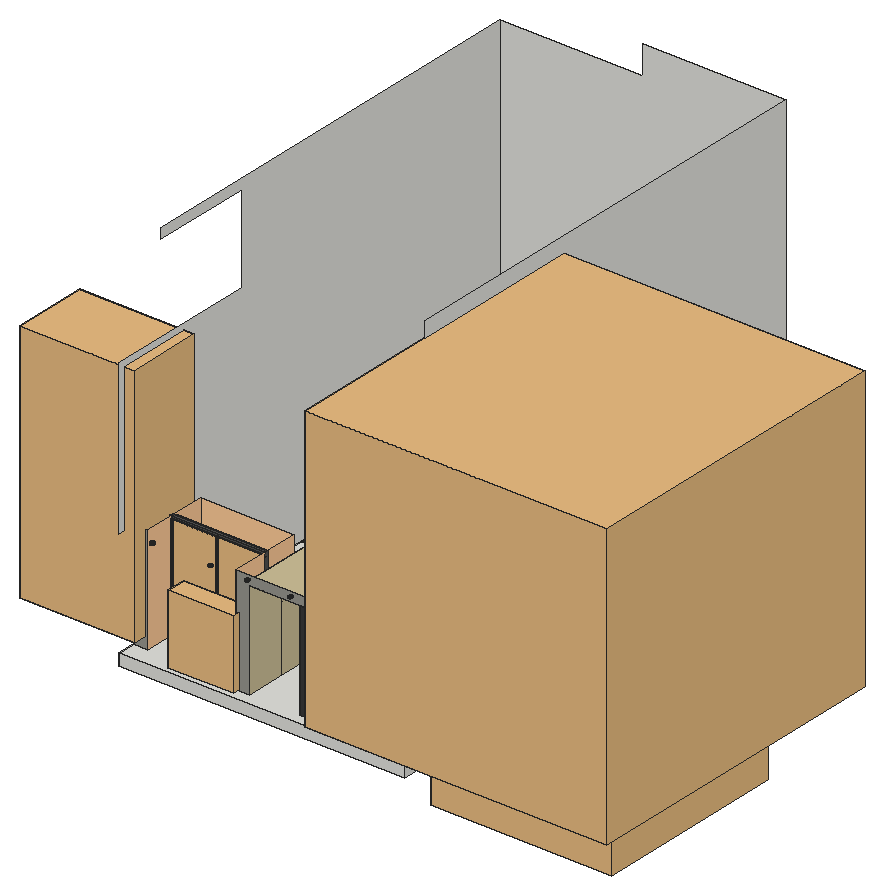
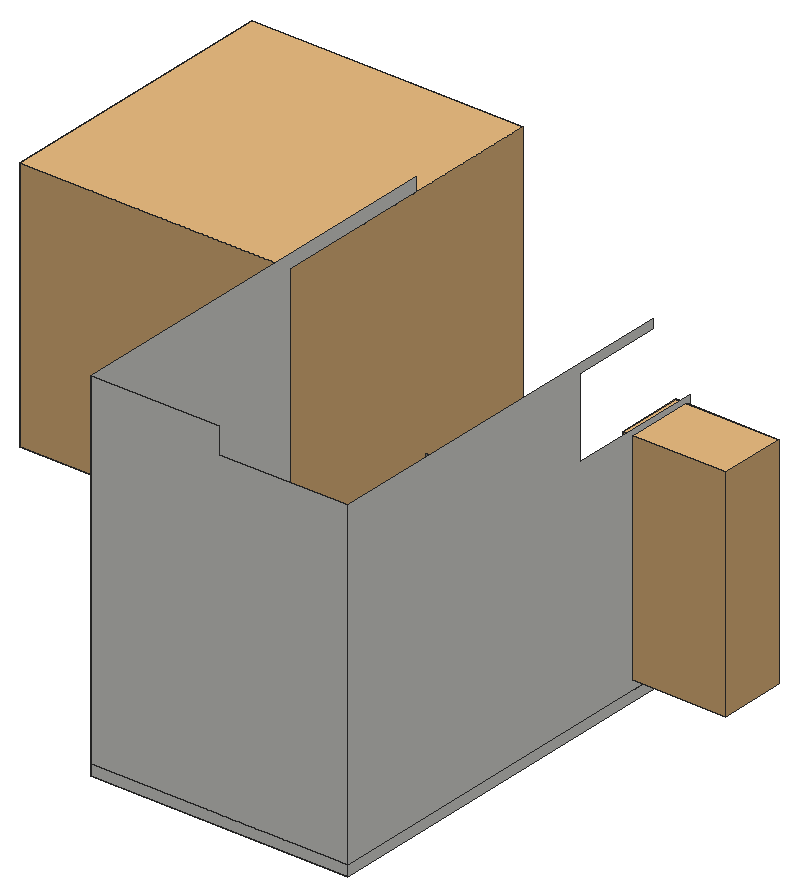
# SketchUp Ruby script. Lengths in inches.
U = 1.inch
M = Sketchup.active_model
def pt(a) = Geom::Point3d.new(a.map { |v| v * U })
def face(e, loops, mat)
  f = e.add_face(loops[0].map { |a| pt(a) })
  loops[1..].each { |l| e.add_face(l.map { |a| pt(a) }).erase! }
  f.material = f.back_material = mat if mat
  f
end
# faces: each face lists its corners as indices into pts; further lists are holes
def faces(e, pts, list, mat = nil) = list.each { |f| face(e, (f[0].is_a?(Array) ? f : [f]).map { |l| l.map { |i| pts[i] } }, mat) }
# xy, xz, yz: faces in a plane at the given z, y or x. An outline is a flat list of corners, or four numbers for a rectangle; further outlines are holes
def ring(l) = l.size == 4 ? [[l[0], l[1]], [l[2], l[1]], [l[2], l[3]], [l[0], l[3]]] : l.each_slice(2).to_a
def flat(e, list, mat, &to3) = list.each { |f| face(e, (f[0].is_a?(Array) ? f : [f]).map { |l| ring(l).map { |u, v| to3.(u, v) } }, mat) }
def xy(e, z, list, mat = nil) = flat(e, list, mat) { |x, y| [x, y, z] }
def xz(e, y, list, mat = nil) = flat(e, list, mat) { |x, z| [x, y, z] }
def yz(e, x, list, mat = nil) = flat(e, list, mat) { |y, z| [x, y, z] }
def lines(e, pts, list) = list.each { |a, b| e.add_line(pt(pts[a]), pt(pts[b])) }
# prism: a flat outline (further loops are holes) pulled along v
def prism(e, loops, v, mat = nil)
  f = face(e, loops, mat); d = Geom::Vector3d.new(v.map { |x| x * U })
  f.pushpull(f.normal.samedirection?(d) ? d.length : -d.length)
end
def box(e, o, s, mat = nil) = prism(e, [[o, [o[0] + s[0], o[1], o[2]], [o[0] + s[0], o[1] + s[1], o[2]], [o[0], o[1] + s[1], o[2]]]], [0, 0, s[2]], mat)
def at(x, y, z, deg = 0) = Geom::Transformation.translation(pt([x, y, z])) * Geom::Transformation.rotation(ORIGIN, Z_AXIS, deg.degrees)
def axes(o, x, y, z) = Geom::Transformation.new([*x, 0, *y, 0, *z, 0, *pt(o).to_a, 1])
def part(name) = M.definitions.add(name)
# library, detail: a bought-in or finely detailed component or shape, given as its bounding box
def library(name, o, s) = part(name).tap { |d| box(d.entities, o, s) }
def detail(e, o, s) = box(e.add_group.entities, o, s)
def put(e, d, t, mat = nil) = e.add_instance(d, t).tap { |i| i.material = mat if mat }
def group(e, t, mat = nil) = e.add_group.tap { |g| g.transformation = t; g.material = mat if mat }.entities
root = M.entities
M.materials.add("AM113_062_Tilia").color = [58, 81, 37]
M.materials.add("AM113_062_Tilia_Bark").color = [88, 85, 72]
M.materials.add("Brick Wall Grey Stone 01 200cm").color = [152, 151, 144]
M.materials.add("Generic").color = [218, 205, 180]
M.materials.add("Glass_Tinted_Gray").color = [0, 0, 0]
M.materials["Glass_Tinted_Gray"].alpha = 0.125
M.materials.add("Wall  Paint Fine Grain 01 Yellow 100cm").color = [207, 193, 153]
M.materials.add("[0135_DarkGray]").color = [81, 81, 81]
M.materials.add("[Color C02]").color = [255, 204, 153]
M.materials.add("[Color E05]").color = [239, 239, 0]
M.materials["[Color E05]"].alpha = 0.89
M.materials.add("[Color M07]").color = [58, 58, 58]
M.materials.add("[Color M08]").color = [30, 30, 30]
M.materials.add("[Granite Dark Gray]").color = [69, 68, 68]
M.materials.add("[Mirror 02]").color = [229, 229, 229]
M.materials.add("[Terrazzo Light Blue]").color = [196, 214, 227]
M.materials.add("[Translucent Glass Gray]").color = [128, 128, 128]
M.materials["[Translucent Glass Gray]"].alpha = 0.5
c1 = library("Curtain set",[0,0,0],[14.46,147.43,135.83])
c2 = part("PENTEK_RP Fineline 50S_Sliding_DoorCase_E1")
box(c2.entities,[0,0,0],[1.51,3.66,99.27],"[0135_DarkGray]")
c3 = part("PENTEK_RP Fineline 50S_SlidingDooe_Case_E2")
box(c3.entities,[0,0,0],[96.25,3.66,1.51],"[0135_DarkGray]")
c4 = part("pentek_RP Fineline 50S_SlidingDoor_Case")
put(c4.entities,c2,at(97.76,0,0))
put(c4.entities,c3,at(1.51,0,0))
put(c4.entities,c2,at(0,0,0))
put(c4.entities,c3,at(1.51,0,97.76))
c5 = part("PENTEK_RP Fineline 50S_SlidingDoor_GlazingBead_2")
box(c5.entities,[0,0,0],[0.56,0.59,94.39],"[0135_DarkGray]")
c6 = part("PENTEK_RP Fineline 50S_SlidingDoor_Glass")
box(c6.entities,[0,0,0],[46.58,0.16,94.39],"Glass_Tinted_Gray")
c7 = part("PENTEK_RP Fineline 50S_SlidingDoor_GlazingBead")
box(c7.entities,[0,0,0],[45.47,0.59,0.56],"[0135_DarkGray]")
c8 = part("PENTEK_RP Fineline 50S_SlidingDoor_Leaf_E1")
xy(c8.entities,0,[[0,0,0.93,1.97],[0.93,1.57,1.49,1.97]],"[0135_DarkGray]")
xy(c8.entities,96.25,[[0,0,0.93,0,0.93,1.57,1.49,1.57,1.49,1.97,0,1.97]],"[0135_DarkGray]")
xz(c8.entities,0,[[0,0,0.93,96.25]],"[0135_DarkGray]")
xz(c8.entities,1.57,[[0.93,0,1.49,95.32],[0.93,95.32,1.49,96.25]],"[0135_DarkGray]")
xz(c8.entities,1.97,[[0,0,1.49,96.25]],"[0135_DarkGray]")
yz(c8.entities,0,[[0,0,1.97,96.25]],"[0135_DarkGray]")
yz(c8.entities,0.93,[[0,0,1.57,0.93],[0,0.93,1.57,95.32],[0,95.32,1.57,96.25]],"[0135_DarkGray]")
yz(c8.entities,1.49,[[1.57,0,1.97,95.32],[1.57,95.32,1.97,96.25]],"[0135_DarkGray]")
c9 = part("PENTEK_RP Fineline 50S_SlidingDoor_Leaf_E2")
xy(c9.entities,0,[[0,0,0,1.57,0.56,1.57,0.56,1.97,46.02,1.97,46.02,1.57,46.58,1.57,46.58,0]],"[0135_DarkGray]")
xy(c9.entities,0.93,[[0,0,46.58,1.57]],"[0135_DarkGray]")
xy(c9.entities,1.49,[[0.56,1.57,46.02,1.97]],"[0135_DarkGray]")
xz(c9.entities,0,[[0,0,46.58,0.93]],"[0135_DarkGray]")
xz(c9.entities,1.57,[[0,0,0.56,0.93],[46.02,0,46.58,0.93],[0.56,0.93,46.02,1.49]],"[0135_DarkGray]")
xz(c9.entities,1.97,[[0.56,0,46.02,1.49]],"[0135_DarkGray]")
yz(c9.entities,0,[[0,0,1.57,0.93]],"[0135_DarkGray]")
yz(c9.entities,0.56,[[1.57,0,1.97,0.93],[1.57,0.93,1.97,1.49]],"[0135_DarkGray]")
yz(c9.entities,46.02,[[1.57,0,1.97,0.93],[1.57,0.93,1.97,1.49]],"[0135_DarkGray]")
yz(c9.entities,46.58,[[0,0,1.57,0.93]],"[0135_DarkGray]")
c10 = part("PENTEK_RP Fineline S_SlidingDoor_Leaf1")
put(c10.entities,c5,at(0.93,0,0.93))
put(c10.entities,c5,at(46.96,0,0.93))
put(c10.entities,c6,at(1.49,1.42,0.93))
put(c10.entities,c7,at(1.49,0,0.93))
put(c10.entities,c6,at(1.49,0.59,0.93),"[Terrazzo Light Blue]")
put(c10.entities,c8,at(0,0,0))
put(c10.entities,c8,axes([48.44,0,0],[-1,0,0],[0,1,0],[0,0,1]))
put(c10.entities,c9,axes([0.93,0,96.25],[1,0,0],[0,1,0],[0,0,-1]))
put(c10.entities,c9,at(0.93,0,0))
put(c10.entities,c7,at(1.49,0,94.77))
c11 = part("PENTEK_RP Fineline 50S_SlidingDoor_Leaf2")
put(c11.entities,c6,at(1.49,1.42,0.93))
put(c11.entities,c7,at(1.49,0,94.77))
put(c11.entities,c5,at(46.96,0,0.93))
put(c11.entities,c6,at(1.49,0.59,0.93),"[Mirror 02]")
put(c11.entities,c5,at(0.93,0,0.93))
put(c11.entities,c8,at(0,0,0))
put(c11.entities,c8,axes([48.44,0,0],[-1,0,0],[0,1,0],[0,0,1]))
put(c11.entities,c7,at(1.49,0,0.93))
put(c11.entities,c9,axes([0.93,0,96.25],[1,0,0],[0,1,0],[0,0,-1]))
put(c11.entities,c9,at(0.93,0,0))
c12 = part("PENTEK - Slimmest Steel Sliding Door / Window\#1")
put(c12.entities,c4,at(0,-1.88,-0.09))
put(c12.entities,c10,at(1.51,-2.27,1.42))
put(c12.entities,c11,at(49.32,-0.3,1.42))
c13 = part("Agrupar\#57")
prism(c13.entities,[[[1.18,24.41,51.97],[1.18,0,51.97],[1.18,0,0],[1.18,24.41,0]],[[1.18,1.57,50.39],[1.18,22.83,50.39],[1.18,22.83,1.57],[1.18,1.57,1.57]]],[-1.18,0,0])
c14 = part("Agrupar\#59")
box(c14.entities,[0,0,0],[0.24,21.26,16.54])
c15 = part("Agrupar\#58")
prism(c15.entities,[[[0,0,0],[0,0,19.69],[0,24.41,19.69],[0,24.41,0]],[[0,1.57,1.57],[0,22.83,1.57],[0,22.83,18.11],[0,1.57,18.11]]],[1.18,0,0])
c16 = part("Agrupar\#56")
box(c16.entities,[0,0,0],[4.72,24.41,1.57])
c17 = part("Agrupar\#55")
prism(c17.entities,[[[0,0,0],[0,0,97.64],[0,27.56,97.64],[0,27.56,0]],[[0,25.98,1.57],[0,25.98,96.0625],[0,1.57,96.0625],[0,1.57,1.57]]],[4.72,0,0])
c18 = part("Agrupar\#60")
box(c18.entities,[0,0,0],[0.24,21.26,48.82])
c19 = part("Janela Maxim ar")
put(c19.entities,c13,at(1.77,1.57,22.83))
put(c19.entities,c14,at(2.36,3.15,77.95),"[Translucent Glass Gray]")
put(c19.entities,c15,at(1.77,1.57,1.57))
put(c19.entities,c16,at(0,1.57,74.8))
put(c19.entities,c16,at(0,1.57,21.26))
put(c19.entities,c15,at(1.77,1.57,76.38))
put(c19.entities,c17,at(0,0,0))
put(c19.entities,c14,at(2.36,3.15,3.15),"[Translucent Glass Gray]")
put(c19.entities,c18,at(2.36,3.15,24.41),"[Translucent Glass Gray]")
c20 = part("Agrupar\#54")
box(c20.entities,[0,0,0],[7.09,27.56,0.79])
c21 = part("JA-70x250")
put(c21.entities,c19,at(2.36,0,0.79),"[Color M08]")
put(c21.entities,c20,at(0,0,0),"[Granite Dark Gray]")
c22 = library("Entrance door assembly",[0,0,0],[51.57,9.61,84.84])
c23 = library("Plant",[-27.84,-31.84,-1.26],[68.28,70.82,154.38])
c24 = library("Group\#7",[0,0,0],[99.27,8.68,96.02])
c25 = library("30",[-486.49,477.14,411.4],[26.62,27.13,73.11])
c26 = library("AM113_062_Tilia_Defintion",[-350.67,-364.73,-2.58],[672.29,726.36,1000])
c27 = library("AM113_062_Tilia_Defintion1",[-524.84,-500,219.37],[933.41,1000,877.77])
c28 = part("Group4\#2")
put(c28.entities,c26,axes([0,0,0],[0.28109,0,0],[0,0.28109,0],[0,0,0.28109]),"AM113_062_Tilia_Bark")
put(c28.entities,c27,axes([0,0,0],[0.33697,0,0],[0,0.33697,0],[0,0,0.33697]),"AM113_062_Tilia")
c29 = part("11")
put(c29.entities,c28,at(1388.71,2.74,19.08))
xy(root,0,[[179.7,11.0625,179.7,207.1875,126.76,207.1875,126.76,54.0625,112.5,54.0625,112.5,88.375,14.7,88.375,14.7,19.125,0,19.125,0,497,299.0625,497,299.0625,12.5,280.68,12.5,280.68,190.6875,189.32,190.6875,189.32,11.0625],[112.5,12.5,126.76,54.0625]])
xy(root,98.74,[[189.32,64.65,280.68,67.0625],[189.32,68.5625,280.68,84.21]])
xy(root,98.74,[[189.32,67.0625,280.68,68.5625]],"[Color E05]")
xy(root,102.36,[[179.7,11.0625,189.32,12.5],[126.76,12.5,179.7,17.9375],[179.7,12.5,189.32,17.9375],[189.32,12.5,280.68,15.9375]])
xy(root,102.36,[[189.32,15.9375,280.68,17.9375]],"[Color E05]")
xy(root,107.49,[[189.32,17.9375,280.68,64.65],[189.32,84.21,280.68,190.6875]])
xy(root,107.49,[[126.76,17.9375,179.7,207.1875]],"Wall  Paint Fine Grain 01 Yellow 100cm")
xy(root,109.8125,[[29.97,4.05,29.45,4.11,28.97,4.3125,28.55,4.63,28.23,5.05,28.03,5.53,27.97,6.05,28.03,6.5625,28.23,7.05,28.55,7.46,28.97,7.78,29.45,7.98,29.97,8.05,30.48,7.98,30.97,7.78,31.38,7.46,31.7,7.05,31.9,6.5625,31.97,6.05,31.9,5.53,31.7,5.05,31.38,4.63,30.97,4.3125,30.48,4.11]])
xy(root,110.68,[[90.97,4.05,90.45,4.11,89.97,4.3125,89.55,4.63,89.23,5.05,89.03,5.53,88.97,6.05,89.03,6.5625,89.23,7.05,89.55,7.46,89.97,7.78,90.45,7.98,90.97,8.05,91.48,7.98,91.97,7.78,92.38,7.46,92.7,7.05,92.9,6.5625,92.97,6.05,92.9,5.53,92.7,5.05,92.38,4.63,91.97,4.3125,91.48,4.11],[129.28,4.05,128.76,4.11,128.28,4.3125,127.86,4.63,127.55,5.05,127.35,5.53,127.28,6.05,127.35,6.5625,127.55,7.05,127.86,7.46,128.28,7.78,128.76,7.98,129.28,8.05,129.8,7.98,130.28,7.78,130.69,7.46,131.01,7.05,131.21,6.5625,131.28,6.05,131.21,5.53,131.01,5.05,130.69,4.63,130.28,4.3125,129.8,4.11],[174.28,4.05,173.76,4.11,173.28,4.3125,172.86,4.63,172.55,5.05,172.35,5.53,172.28,6.05,172.35,6.5625,172.55,7.05,172.86,7.46,173.28,7.78,173.76,7.98,174.28,8.05,174.8,7.98,175.28,7.78,175.69,7.46,176.01,7.05,176.21,6.5625,176.28,6.05,176.21,5.53,176.01,5.05,175.69,4.63,175.28,4.3125,174.8,4.11],[208.4,4.05,207.89,4.11,207.4,4.3125,206.99,4.63,206.67,5.05,206.47,5.53,206.4,6.05,206.47,6.5625,206.67,7.05,206.99,7.46,207.4,7.78,207.89,7.98,208.4,8.05,208.92,7.98,209.4,7.78,209.82,7.46,210.14,7.05,210.34,6.5625,210.4,6.05,210.34,5.53,210.14,5.05,209.82,4.63,209.4,4.3125,208.92,4.11],[237.34,4.05,236.82,4.11,236.34,4.3125,235.93,4.63,235.61,5.05,235.41,5.53,235.34,6.05,235.41,6.5625,235.61,7.05,235.93,7.46,236.34,7.78,236.82,7.98,237.34,8.05,237.86,7.98,238.34,7.78,238.76,7.46,239.07,7.05,239.27,6.5625,239.34,6.05,239.27,5.53,239.07,5.05,238.76,4.63,238.34,4.3125,237.86,4.11],
  [267.84,4.05,267.32,4.11,266.84,4.3125,266.43,4.63,266.11,5.05,265.91,5.53,265.84,6.05,265.91,6.5625,266.11,7.05,266.43,7.46,266.84,7.78,267.32,7.98,267.84,8.05,268.36,7.98,268.84,7.78,269.26,7.46,269.57,7.05,269.77,6.5625,269.84,6.05,269.77,5.53,269.57,5.05,269.26,4.63,268.84,4.3125,268.36,4.11]])
xz(root,11.0625,[[179.7,0,189.32,102.36]],"[Color M07]")
xz(root,12.5,[[112.5,0,126.76,0,126.76,102.36,280.68,102.36,280.68,0,299.0625,0,299.0625,111.61,112.5,111.61]],"Brick Wall Grey Stone 01 200cm")
xz(root,17.9375,[[126.76,102.36,179.7,107.49],[179.7,102.36,189.32,107.49],[189.32,102.36,280.68,107.49]])
xz(root,19.125,[[0,0,14.7,111.61]],"Brick Wall Grey Stone 01 200cm")
xz(root,64.65,[[189.32,98.74,280.68,107.49]])
xz(root,84.21,[[189.32,98.74,280.68,107.49]])
xz(root,88.375,[[14.7,0,112.5,111.61]],"[Color C02]")
xz(root,190.6875,[[189.32,0,280.68,107.49]],"Generic")
xz(root,207.1875,[[126.76,0,179.7,107.49]])
xz(root,497,[[0,0,0,374.3125,149.53,374.3125,149.53,404.5625,299.0625,404.5625,299.0625,0]])
yz(root,0,[[19.125,0,19.125,111.61,0,111.61,0,271.39,159.875,271.39,159.875,363.53,54.0625,363.53,54.0625,374.3125,497,374.3125,497,0]])
yz(root,14.7,[[19.125,0,88.375,111.61]],"[Color C02]")
yz(root,112.5,[[12.5,0,88.375,111.61]],"[Color C02]")
yz(root,126.76,[[12.5,0,54.0625,0,54.0625,107.49,17.9375,107.49,17.9375,102.36,12.5,102.36],[54.0625,0,207.1875,107.49]],"Wall  Paint Fine Grain 01 Yellow 100cm")
yz(root,179.7,[[11.0625,0,11.0625,102.36,17.9375,102.36,17.9375,107.49,207.1875,107.49,207.1875,0]],"Wall  Paint Fine Grain 01 Yellow 100cm")
yz(root,189.32,[[11.0625,0,64.65,0,64.65,107.49,17.9375,107.49,17.9375,102.36,11.0625,102.36]])
yz(root,189.32,[[64.65,0,190.6875,0,190.6875,107.49,84.21,107.49,84.21,98.74,64.65,98.74]],"Generic")
yz(root,280.68,[[12.5,0,15.9375,102.36],[17.9375,0,64.65,107.49]])
yz(root,280.68,[[64.65,0,64.65,98.74,84.21,98.74,84.21,107.49,190.6875,107.49,190.6875,0]],"Generic")
yz(root,280.68,[[15.9375,0,17.9375,102.36]],"[Color E05]")
yz(root,299.0625,[[12.5,0,497,0,497,404.5625,25.125,404.5625,25.125,120,0,120,0,111.61,12.5,111.61]])
p = [[29.97,4.05,111.61],[29.45,4.11,111.61],[29.45,4.11,109.8125],[29.97,4.05,109.8125],[30.48,4.11,111.61],[30.48,4.11,109.8125],
  [28.97,4.3125,111.61],[28.97,4.3125,109.8125],[30.97,4.3125,111.61],[30.97,4.3125,109.8125],[28.55,4.63,111.61],[28.55,4.63,109.8125],
  [31.38,4.63,111.61],[31.38,4.63,109.8125],[28.23,5.05,111.61],[28.23,5.05,109.8125],[31.7,5.05,111.61],[31.7,5.05,109.8125],
  [28.03,5.53,111.61],[28.03,5.53,109.8125],[31.9,5.53,111.61],[31.9,5.53,109.8125],[27.97,6.05,111.61],[27.97,6.05,109.8125],
  [31.97,6.05,111.61],[31.97,6.05,109.8125],[28.03,6.5625,111.61],[28.03,6.5625,109.8125],[31.9,6.5625,111.61],[31.9,6.5625,109.8125],
  [28.23,7.05,111.61],[28.23,7.05,109.8125],[31.7,7.05,111.61],[31.7,7.05,109.8125],[28.55,7.46,111.61],[28.55,7.46,109.8125],
  [31.38,7.46,111.61],[31.38,7.46,109.8125],[28.97,7.78,111.61],[28.97,7.78,109.8125],[30.97,7.78,111.61],[30.97,7.78,109.8125],
  [29.45,7.98,111.61],[29.45,7.98,109.8125],[30.48,7.98,111.61],[30.48,7.98,109.8125],[29.97,8.05,111.61],[29.97,8.05,109.8125],
  [90.97,4.05,111.61],[90.45,4.11,111.61],[90.45,4.11,110.68],[90.97,4.05,110.68],[91.48,4.11,111.61],[91.48,4.11,110.68],
  [129.28,4.05,111.61],[128.76,4.11,111.61],[128.76,4.11,110.68],[129.28,4.05,110.68],[129.8,4.11,111.61],[129.8,4.11,110.68],
  [174.28,4.05,111.61],[173.76,4.11,111.61],[173.76,4.11,110.68],[174.28,4.05,110.68],[174.8,4.11,111.61],[174.8,4.11,110.68],
  [208.4,4.05,111.61],[207.89,4.11,111.61],[207.89,4.11,110.68],[208.4,4.05,110.68],[208.92,4.11,111.61],[208.92,4.11,110.68],
  [237.34,4.05,111.61],[236.82,4.11,111.61],[236.82,4.11,110.68],[237.34,4.05,110.68],[237.86,4.11,111.61],[237.86,4.11,110.68],
  [267.84,4.05,111.61],[267.32,4.11,111.61],[267.32,4.11,110.68],[267.84,4.05,110.68],[268.36,4.11,111.61],[268.36,4.11,110.68],
  [89.97,4.3125,111.61],[89.97,4.3125,110.68],[91.97,4.3125,111.61],[91.97,4.3125,110.68],[128.28,4.3125,111.61],[128.28,4.3125,110.68],
  [130.28,4.3125,111.61],[130.28,4.3125,110.68],[173.28,4.3125,111.61],[173.28,4.3125,110.68],[175.28,4.3125,111.61],[175.28,4.3125,110.68],
  [207.4,4.3125,111.61],[207.4,4.3125,110.68],[209.4,4.3125,111.61],[209.4,4.3125,110.68],[236.34,4.3125,111.61],[236.34,4.3125,110.68],
  [238.34,4.3125,111.61],[238.34,4.3125,110.68],[266.84,4.3125,111.61],[266.84,4.3125,110.68],[268.84,4.3125,111.61],[268.84,4.3125,110.68],
  [89.55,4.63,111.61],[89.55,4.63,110.68],[92.38,4.63,111.61],[92.38,4.63,110.68],[127.86,4.63,111.61],[127.86,4.63,110.68],
  [130.69,4.63,111.61],[130.69,4.63,110.68],[172.86,4.63,111.61],[172.86,4.63,110.68],[175.69,4.63,111.61],[175.69,4.63,110.68],
  [206.99,4.63,111.61],[206.99,4.63,110.68],[209.82,4.63,111.61],[209.82,4.63,110.68],[235.93,4.63,111.61],[235.93,4.63,110.68],
  [238.76,4.63,111.61],[238.76,4.63,110.68],[266.43,4.63,111.61],[266.43,4.63,110.68],[269.26,4.63,111.61],[269.26,4.63,110.68],
  [89.23,5.05,111.61],[89.23,5.05,110.68],[92.7,5.05,111.61],[92.7,5.05,110.68],[127.55,5.05,111.61],[127.55,5.05,110.68],
  [131.01,5.05,111.61],[131.01,5.05,110.68],[172.55,5.05,111.61],[172.55,5.05,110.68],[176.01,5.05,111.61],[176.01,5.05,110.68],
  [206.67,5.05,111.61],[206.67,5.05,110.68],[210.14,5.05,111.61],[210.14,5.05,110.68],[235.61,5.05,111.61],[235.61,5.05,110.68],
  [239.07,5.05,111.61],[239.07,5.05,110.68],[266.11,5.05,111.61],[266.11,5.05,110.68],[269.57,5.05,111.61],[269.57,5.05,110.68],
  [89.03,5.53,111.61],[89.03,5.53,110.68],[92.9,5.53,111.61],[92.9,5.53,110.68],[127.35,5.53,111.61],[127.35,5.53,110.68],
  [131.21,5.53,111.61],[131.21,5.53,110.68],[172.35,5.53,111.61],[172.35,5.53,110.68],[176.21,5.53,111.61],[176.21,5.53,110.68],
  [206.47,5.53,111.61],[206.47,5.53,110.68],[210.34,5.53,111.61],[210.34,5.53,110.68],[235.41,5.53,111.61],[235.41,5.53,110.68],
  [239.27,5.53,111.61],[239.27,5.53,110.68],[265.91,5.53,111.61],[265.91,5.53,110.68],[269.77,5.53,111.61],[269.77,5.53,110.68],
  [88.97,6.05,111.61],[88.97,6.05,110.68],[92.97,6.05,111.61],[92.97,6.05,110.68],[127.28,6.05,111.61],[127.28,6.05,110.68],
  [131.28,6.05,111.61],[131.28,6.05,110.68],[172.28,6.05,111.61],[172.28,6.05,110.68],[176.28,6.05,111.61],[176.28,6.05,110.68],
  [206.4,6.05,111.61],[206.4,6.05,110.68],[210.4,6.05,111.61],[210.4,6.05,110.68],[235.34,6.05,111.61],[235.34,6.05,110.68],
  [239.34,6.05,111.61],[239.34,6.05,110.68],[265.84,6.05,111.61],[265.84,6.05,110.68],[269.84,6.05,111.61],[269.84,6.05,110.68],
  [89.03,6.5625,111.61],[89.03,6.5625,110.68],[92.9,6.5625,111.61],[92.9,6.5625,110.68],[127.35,6.5625,111.61],[127.35,6.5625,110.68],
  [131.21,6.5625,111.61],[131.21,6.5625,110.68],[172.35,6.5625,111.61],[172.35,6.5625,110.68],[176.21,6.5625,111.61],[176.21,6.5625,110.68],
  [206.47,6.5625,111.61],[206.47,6.5625,110.68],[210.34,6.5625,111.61],[210.34,6.5625,110.68],[235.41,6.5625,111.61],[235.41,6.5625,110.68],
  [239.27,6.5625,111.61],[239.27,6.5625,110.68],[265.91,6.5625,111.61],[265.91,6.5625,110.68],[269.77,6.5625,111.61],[269.77,6.5625,110.68],
  [89.23,7.05,111.61],[89.23,7.05,110.68],[92.7,7.05,111.61],[92.7,7.05,110.68],[127.55,7.05,111.61],[127.55,7.05,110.68],
  [131.01,7.05,111.61],[131.01,7.05,110.68],[172.55,7.05,111.61],[172.55,7.05,110.68],[176.01,7.05,111.61],[176.01,7.05,110.68],
  [206.67,7.05,111.61],[206.67,7.05,110.68],[210.14,7.05,111.61],[210.14,7.05,110.68],[235.61,7.05,111.61],[235.61,7.05,110.68],
  [239.07,7.05,111.61],[239.07,7.05,110.68],[266.11,7.05,111.61],[266.11,7.05,110.68],[269.57,7.05,111.61],[269.57,7.05,110.68],
  [89.55,7.46,111.61],[89.55,7.46,110.68],[92.38,7.46,111.61],[92.38,7.46,110.68],[127.86,7.46,111.61],[127.86,7.46,110.68],
  [130.69,7.46,111.61],[130.69,7.46,110.68],[172.86,7.46,111.61],[172.86,7.46,110.68],[175.69,7.46,111.61],[175.69,7.46,110.68],
  [206.99,7.46,111.61],[206.99,7.46,110.68],[209.82,7.46,111.61],[209.82,7.46,110.68],[235.93,7.46,111.61],[235.93,7.46,110.68],
  [238.76,7.46,111.61],[238.76,7.46,110.68],[266.43,7.46,111.61],[266.43,7.46,110.68],[269.26,7.46,111.61],[269.26,7.46,110.68],
  [89.97,7.78,111.61],[89.97,7.78,110.68],[91.97,7.78,111.61],[91.97,7.78,110.68],[128.28,7.78,111.61],[128.28,7.78,110.68],
  [130.28,7.78,111.61],[130.28,7.78,110.68],[173.28,7.78,111.61],[173.28,7.78,110.68],[175.28,7.78,111.61],[175.28,7.78,110.68],
  [207.4,7.78,111.61],[207.4,7.78,110.68],[209.4,7.78,111.61],[209.4,7.78,110.68],[236.34,7.78,111.61],[236.34,7.78,110.68],
  [238.34,7.78,111.61],[238.34,7.78,110.68],[266.84,7.78,111.61],[266.84,7.78,110.68],[268.84,7.78,111.61],[268.84,7.78,110.68],
  [90.45,7.98,111.61],[90.45,7.98,110.68],[91.48,7.98,111.61],[91.48,7.98,110.68],[128.76,7.98,111.61],[128.76,7.98,110.68],
  [129.8,7.98,111.61],[129.8,7.98,110.68],[173.76,7.98,111.61],[173.76,7.98,110.68],[174.8,7.98,111.61],[174.8,7.98,110.68],
  [207.89,7.98,111.61],[207.89,7.98,110.68],[208.92,7.98,111.61],[208.92,7.98,110.68],[236.82,7.98,111.61],[236.82,7.98,110.68],
  [237.86,7.98,111.61],[237.86,7.98,110.68],[267.32,7.98,111.61],[267.32,7.98,110.68],[268.36,7.98,111.61],[268.36,7.98,110.68],
  [90.97,8.05,111.61],[90.97,8.05,110.68],[129.28,8.05,111.61],[129.28,8.05,110.68],[174.28,8.05,111.61],[174.28,8.05,110.68],
  [208.4,8.05,111.61],[208.4,8.05,110.68],[237.34,8.05,111.61],[237.34,8.05,110.68],[267.84,8.05,111.61],[267.84,8.05,110.68]]
faces(root,p,[[0,1,2,3],[4,0,3,5],[1,6,7,2],[8,4,5,9],[6,10,11,7],[12,8,9,13],[10,14,15,11],[16,12,13,17],
  [14,18,19,15],[20,16,17,21],[18,22,23,19],[24,20,21,25],[22,26,27,23],[28,24,25,29],[26,30,31,27],[32,28,29,33],
  [30,34,35,31],[36,32,33,37],[34,38,39,35],[40,36,37,41],[38,42,43,39],[44,40,41,45],[42,46,47,43],[46,44,45,47],
  [48,49,50,51],[52,48,51,53],[54,55,56,57],[58,54,57,59],[60,61,62,63],[64,60,63,65],[66,67,68,69],[70,66,69,71],
  [72,73,74,75],[76,72,75,77],[78,79,80,81],[82,78,81,83],[49,84,85,50],[86,52,53,87],[55,88,89,56],[90,58,59,91],
  [61,92,93,62],[94,64,65,95],[67,96,97,68],[98,70,71,99],[73,100,101,74],[102,76,77,103],[79,104,105,80],[106,82,83,107],
  [84,108,109,85],[110,86,87,111],[88,112,113,89],[114,90,91,115],[92,116,117,93],[118,94,95,119],[96,120,121,97],[122,98,99,123],
  [100,124,125,101],[126,102,103,127],[104,128,129,105],[130,106,107,131],[108,132,133,109],[134,110,111,135],[112,136,137,113],[138,114,115,139],
  [116,140,141,117],[142,118,119,143],[120,144,145,121],[146,122,123,147],[124,148,149,125],[150,126,127,151],[128,152,153,129],[154,130,131,155],
  [132,156,157,133],[158,134,135,159],[136,160,161,137],[162,138,139,163],[140,164,165,141],[166,142,143,167],[144,168,169,145],[170,146,147,171],
  [148,172,173,149],[174,150,151,175],[152,176,177,153],[178,154,155,179],[156,180,181,157],[182,158,159,183],[160,184,185,161],[186,162,163,187],
  [164,188,189,165],[190,166,167,191],[168,192,193,169],[194,170,171,195],[172,196,197,173],[198,174,175,199],[176,200,201,177],[202,178,179,203],
  [180,204,205,181],[206,182,183,207],[184,208,209,185],[210,186,187,211],[188,212,213,189],[214,190,191,215],[192,216,217,193],[218,194,195,219],
  [196,220,221,197],[222,198,199,223],[200,224,225,201],[226,202,203,227],[204,228,229,205],[230,206,207,231],[208,232,233,209],[234,210,211,235],
  [212,236,237,213],[238,214,215,239],[216,240,241,217],[242,218,219,243],[220,244,245,221],[246,222,223,247],[224,248,249,225],[250,226,227,251],
  [228,252,253,229],[254,230,231,255],[232,256,257,233],[258,234,235,259],[236,260,261,237],[262,238,239,263],[240,264,265,241],[266,242,243,267],
  [244,268,269,245],[270,246,247,271],[248,272,273,249],[274,250,251,275],[252,276,277,253],[278,254,255,279],[256,280,281,257],[282,258,259,283],
  [260,284,285,261],[286,262,263,287],[264,288,289,265],[290,266,267,291],[268,292,293,269],[294,270,271,295],[272,296,297,273],[298,274,275,299],
  [276,300,301,277],[302,278,279,303],[280,304,305,281],[306,282,283,307],[284,308,309,285],[310,286,287,311],[288,312,313,289],[314,290,291,315],
  [292,316,317,293],[318,294,295,319],[296,320,321,297],[322,298,299,323],[300,324,325,301],[324,302,303,325],[304,326,327,305],[326,306,307,327],
  [308,328,329,309],[328,310,311,329],[312,330,331,313],[330,314,315,331],[316,332,333,317],[332,318,319,333],[320,334,335,321],[334,322,323,335]])
g1 = group(root,at(0,497,-12.0625))
box(g1,[0,-497,0],[299.0625,497,12.0625])
put(root,c1,axes([110.06,49.56,-3.01],[0,0.6,0],[-0.64653,0,0],[0,0,0.822]))
put(root,c12,axes([13.23,51.83,0.1],[1,0,0],[0,1,0],[0,0,1.12431]))
put(root,c21,at(0,54.0625,0))
put(root,c22,axes([132.625,196.37,0],[0.8352,0,0],[0,-0.3,0],[0,0,1]))
put(root,c23,axes([74.48,15.31,0.59],[1,0,0],[0,0.2866,0],[0,0,0.46989]))
put(root,c24,at(189.32,83.82,2.72))
put(root,c25,axes([2080.81,-1353.24,-1421.56],[4.5,0,0],[0,2.85,0],[0,0,3.4821]))
put(root,c29,at(-913.3,35.79,0))
